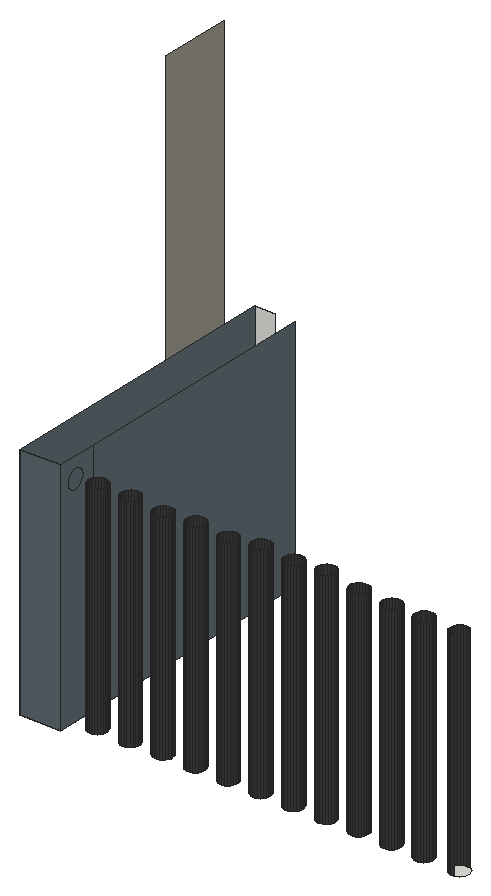
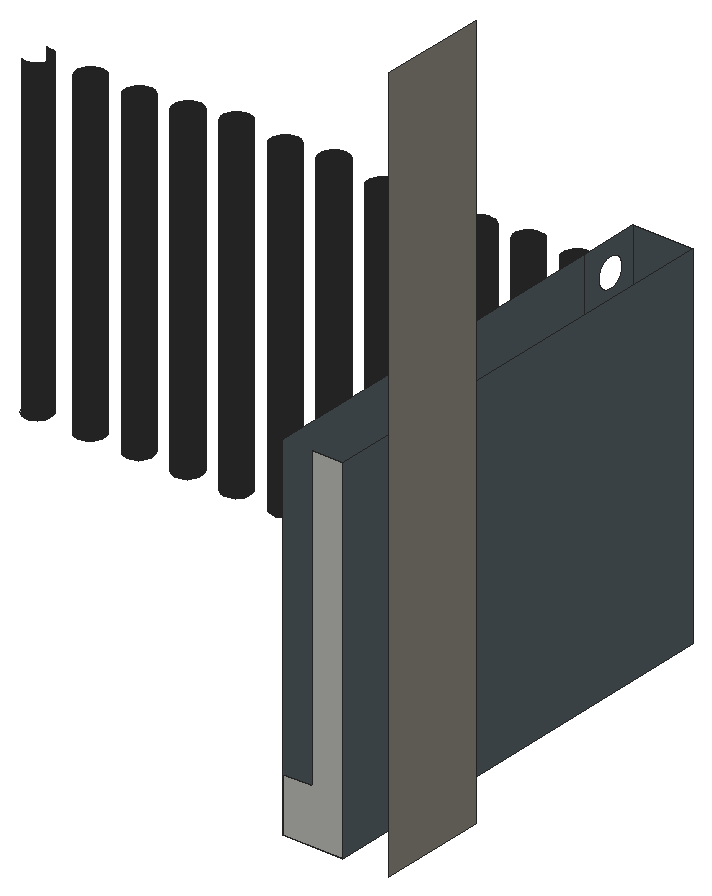
# SketchUp Ruby script. Lengths in inches.
U = 1.inch
M = Sketchup.active_model
def pt(a) = Geom::Point3d.new(a.map { |v| v * U })
def face(e, loops, mat)
  f = e.add_face(loops[0].map { |a| pt(a) })
  loops[1..].each { |l| e.add_face(l.map { |a| pt(a) }).erase! }
  f.material = f.back_material = mat if mat
  f
end
# faces: each face lists its corners as indices into pts; further lists are holes
def faces(e, pts, list, mat = nil) = list.each { |f| face(e, (f[0].is_a?(Array) ? f : [f]).map { |l| l.map { |i| pts[i] } }, mat) }
# xy, xz, yz: faces in a plane at the given z, y or x. An outline is a flat list of corners, or four numbers for a rectangle; further outlines are holes
def ring(l) = l.size == 4 ? [[l[0], l[1]], [l[2], l[1]], [l[2], l[3]], [l[0], l[3]]] : l.each_slice(2).to_a
def flat(e, list, mat, &to3) = list.each { |f| face(e, (f[0].is_a?(Array) ? f : [f]).map { |l| ring(l).map { |u, v| to3.(u, v) } }, mat) }
def xy(e, z, list, mat = nil) = flat(e, list, mat) { |x, y| [x, y, z] }
def xz(e, y, list, mat = nil) = flat(e, list, mat) { |x, z| [x, y, z] }
def yz(e, x, list, mat = nil) = flat(e, list, mat) { |y, z| [x, y, z] }
def lines(e, pts, list) = list.each { |a, b| e.add_line(pt(pts[a]), pt(pts[b])) }
# prism: a flat outline (further loops are holes) pulled along v
def prism(e, loops, v, mat = nil)
  f = face(e, loops, mat); d = Geom::Vector3d.new(v.map { |x| x * U })
  f.pushpull(f.normal.samedirection?(d) ? d.length : -d.length)
end
def box(e, o, s, mat = nil) = prism(e, [[o, [o[0] + s[0], o[1], o[2]], [o[0] + s[0], o[1] + s[1], o[2]], [o[0], o[1] + s[1], o[2]]]], [0, 0, s[2]], mat)
def at(x, y, z, deg = 0) = Geom::Transformation.translation(pt([x, y, z])) * Geom::Transformation.rotation(ORIGIN, Z_AXIS, deg.degrees)
def axes(o, x, y, z) = Geom::Transformation.new([*x, 0, *y, 0, *z, 0, *pt(o).to_a, 1])
def part(name) = M.definitions.add(name)
# library, detail: a bought-in or finely detailed component or shape, given as its bounding box
def library(name, o, s) = part(name).tap { |d| box(d.entities, o, s) }
def detail(e, o, s) = box(e.add_group.entities, o, s)
def put(e, d, t, mat = nil) = e.add_instance(d, t).tap { |i| i.material = mat if mat }
def group(e, t, mat = nil) = e.add_group.tap { |g| g.transformation = t; g.material = mat if mat }.entities
root = M.entities
M.materials.add("[Color M07]").color = [58, 58, 58]
M.materials.add("[Formica Graystone]").color = [149, 146, 135]
M.materials.add("[Formica Speckled Grey]").color = [94, 105, 111]
xy(root,452.9,[[220.36,118.22,223.91,144.04],[225.65,119.22,225.45,119.27,225.26,119.375,225.11,119.52,225,119.71,224.94,119.91,224.94,120.125,225,120.33,225.1,120.51,225.25,120.67,225.43,120.77,225.63,120.83,225.85,120.83,226.05,120.78,226.24,120.68,226.39,120.53,226.5,120.35,226.55,120.14,226.56,119.93,226.5,119.72,226.4,119.54,226.25,119.39,226.07,119.28,225.86,119.22],[228.53,119.22,228.32,119.27,228.14,119.375,227.98,119.52,227.875,119.71,227.82,119.91,227.82,120.125,227.87,120.33,227.97,120.51,228.12,120.67,228.3,120.77,228.51,120.83,228.72,120.83,228.93,120.78,229.11,120.68,229.26,120.53,229.37,120.35,229.43,120.14,229.43,119.93,229.38,119.72,229.27,119.54,229.125,119.39,228.94,119.28,228.74,119.22],[231.4,119.22,231.2,119.27,231.01,119.375,230.86,119.52,230.75,119.71,230.69,119.91,230.69,120.125,230.75,120.33,230.85,120.51,231,120.67,231.18,120.77,231.38,120.83,231.6,120.83,231.8,120.78,231.99,120.68,232.14,120.53,232.25,120.35,232.3,120.14,232.31,119.93,232.25,119.72,232.15,119.54,232,119.39,231.82,119.28,231.61,119.22],[234.28,119.22,234.07,119.27,233.89,119.375,233.73,119.52,233.625,119.71,233.57,119.91,233.57,120.125,233.62,120.33,233.72,120.51,233.87,120.67,234.05,120.77,234.26,120.83,234.47,120.83,234.68,120.78,234.86,120.68,235.01,120.53,235.12,120.35,235.18,120.14,235.18,119.93,235.13,119.72,235.02,119.54,234.875,119.39,234.69,119.28,234.49,119.22],
  [237.15,119.22,236.95,119.27,236.76,119.375,236.61,119.52,236.5,119.71,236.44,119.91,236.44,120.125,236.5,120.33,236.6,120.51,236.75,120.67,236.93,120.77,237.13,120.83,237.35,120.83,237.55,120.78,237.74,120.68,237.89,120.53,238,120.35,238.05,120.14,238.06,119.93,238,119.72,237.9,119.54,237.75,119.39,237.57,119.28,237.36,119.22],[240.03,119.22,239.82,119.27,239.64,119.375,239.48,119.52,239.375,119.71,239.32,119.91,239.32,120.125,239.37,120.33,239.47,120.51,239.62,120.67,239.8,120.77,240.01,120.83,240.22,120.83,240.43,120.78,240.61,120.68,240.76,120.53,240.87,120.35,240.93,120.14,240.93,119.93,240.88,119.72,240.77,119.54,240.625,119.39,240.44,119.28,240.24,119.22],[242.9,119.22,242.7,119.27,242.51,119.375,242.36,119.52,242.25,119.71,242.19,119.91,242.19,120.125,242.25,120.33,242.35,120.51,242.5,120.67,242.68,120.77,242.88,120.83,243.1,120.83,243.3,120.78,243.49,120.68,243.64,120.53,243.75,120.35,243.8,120.14,243.81,119.93,243.75,119.72,243.65,119.54,243.5,119.39,243.32,119.28,243.11,119.22],[245.78,119.22,245.57,119.27,245.39,119.375,245.23,119.52,245.125,119.71,245.07,119.91,245.07,120.125,245.12,120.33,245.22,120.51,245.37,120.67,245.55,120.77,245.76,120.83,245.97,120.83,246.18,120.78,246.36,120.68,246.51,120.53,246.62,120.35,246.68,120.14,246.68,119.93,246.63,119.72,246.52,119.54,246.375,119.39,246.19,119.28,245.99,119.22],[248.65,119.22,248.45,119.27,248.26,119.375,248.11,119.52,248,119.71,247.94,119.91,247.94,120.125,248,120.33,248.1,120.51,248.25,120.67,248.43,120.77,248.63,120.83,248.85,120.83,249.05,120.78,249.24,120.68,249.39,120.53,249.5,120.35,249.55,120.14,249.56,119.93,249.5,119.72,249.4,119.54,249.25,119.39,249.07,119.28,248.86,119.22],
  [251.53,119.22,251.32,119.27,251.14,119.375,250.98,119.52,250.875,119.71,250.82,119.91,250.82,120.125,250.87,120.33,250.97,120.51,251.12,120.67,251.3,120.77,251.51,120.83,251.72,120.83,251.93,120.78,252.11,120.68,252.26,120.53,252.37,120.35,252.43,120.14,252.43,119.93,252.38,119.72,252.27,119.54,252.125,119.39,251.94,119.28,251.74,119.22],[254.4,119.22,254.2,119.27,254.01,119.375,253.86,119.52,253.75,119.71,253.69,119.91,253.69,120.125,253.75,120.33,253.85,120.51,254,120.67,254.18,120.77,254.38,120.83,254.6,120.83,254.8,120.78,254.99,120.68,255.14,120.53,255.25,120.35,255.3,120.14,255.31,119.93,255.25,119.72,255.15,119.54,255,119.39,254.82,119.28,254.61,119.22],[257.53,119.22,257.32,119.27,257.14,119.375,256.98,119.52,256.875,119.71,256.82,119.91,256.82,120.125,256.87,120.33,256.97,120.51,257.12,120.67,257.3,120.77,257.51,120.83,257.72,120.83,257.93,120.78,258.11,120.68,258.26,120.53,258.37,120.35,258.43,120.14,258.43,119.93,258.38,119.72,258.27,119.54,258.125,119.39,257.94,119.28,257.74,119.22]])
xz(root,118.22,[[220.36,452.9,223.91,473.83]],"[Formica Speckled Grey]")
xz(root,119.22,[[225.65,452.9,225.86,472.27],[228.53,452.9,228.74,472.27],[231.4,452.9,231.61,472.05],[234.28,452.9,234.49,472.27],[237.15,452.9,237.36,472.05],
  [240.03,452.9,240.24,472.48],[242.9,452.9,243.11,472.27],[245.78,452.9,245.99,472.48],[248.65,452.9,248.86,472.05],[251.53,452.9,251.74,471.82],
  [254.4,452.9,254.61,471.82],[257.53,452.9,257.74,471.82]],"[Color M07]")
xz(root,120.83,[[225.63,452.9,225.85,472.27],[228.51,452.9,228.72,472.27],[231.38,452.9,231.6,472.05],[234.26,452.9,234.47,472.27],[237.13,452.9,237.35,472.05],
  [240.01,452.9,240.22,472.48],[242.88,452.9,243.1,472.27],[245.76,452.9,245.97,472.48],[248.63,452.9,248.85,472.05],[251.51,452.9,251.72,471.82],
  [254.38,452.9,254.6,471.82],[257.51,452.9,257.72,471.82]],"[Color M07]")
xz(root,144.04,[[220.36,452.9,223.91,452.9,223.91,456.09,222.16,456.09,222.16,473.83,220.36,473.83]])
yz(root,217.65,[[137.66,452.9,144.04,495.41]],"[Formica Graystone]")
yz(root,220.36,[[118.22,452.9,144.04,473.83]],"[Formica Speckled Grey]")
yz(root,223.91,[[[118.22,452.9,121.78,473.83],[119.86,471.17,119.64,471.2,119.42,471.29,119.24,471.43,119.1,471.61,119.02,471.82,118.99,472.05,119.02,472.27,119.1,472.48,119.24,472.67,119.42,472.81,119.64,472.89,119.86,472.92,120.09,472.89,120.3,472.81,120.48,472.67,120.62,472.48,120.71,472.27,120.74,472.05,120.71,471.82,120.62,471.61,120.48,471.43,120.3,471.29,120.09,471.2]],[121.78,452.9,144.04,473.83]],"[Formica Speckled Grey]")
yz(root,224.94,[[119.91,452.9,120.125,472.27]],"[Color M07]")
yz(root,227.82,[[119.91,452.9,120.125,472.27]],"[Color M07]")
yz(root,229.43,[[119.93,452.9,120.14,472.27]],"[Color M07]")
yz(root,230.69,[[119.91,452.9,120.125,472.05]],"[Color M07]")
yz(root,233.57,[[119.91,452.9,120.125,472.27]],"[Color M07]")
yz(root,235.18,[[119.93,452.9,120.14,472.27]],"[Color M07]")
yz(root,236.44,[[119.91,452.9,120.125,472.05]],"[Color M07]")
yz(root,239.32,[[119.91,452.9,120.125,472.48]],"[Color M07]")
yz(root,240.93,[[119.93,452.9,120.14,472.48]],"[Color M07]")
yz(root,242.19,[[119.91,452.9,120.125,472.27]],"[Color M07]")
yz(root,245.07,[[119.91,452.9,120.125,472.48]],"[Color M07]")
yz(root,246.68,[[119.93,452.9,120.14,472.48]],"[Color M07]")
yz(root,247.94,[[119.91,452.9,120.125,472.05]],"[Color M07]")
yz(root,250.82,[[119.91,452.9,120.125,471.82]],"[Color M07]")
yz(root,252.43,[[119.93,452.9,120.14,471.82]],"[Color M07]")
yz(root,253.69,[[119.91,452.9,120.125,471.82]],"[Color M07]")
yz(root,256.82,[[119.91,452.9,120.125,471.82]],"[Color M07]")
p = [[225.45,119.27,452.9],[225.65,119.22,452.9],[225.65,119.22,472.27],[225.45,119.27,472.27],[225.86,119.22,452.9],[226.07,119.28,452.9],
  [226.07,119.28,472.27],[225.86,119.22,472.27],[228.32,119.27,452.9],[228.53,119.22,452.9],[228.53,119.22,472.27],[228.32,119.27,472.27],
  [228.74,119.22,452.9],[228.94,119.28,452.9],[228.94,119.28,472.27],[228.74,119.22,472.27],[231.2,119.27,452.9],[231.4,119.22,452.9],
  [231.4,119.22,472.05],[231.2,119.27,472.05],[231.61,119.22,452.9],[231.82,119.28,452.9],[231.82,119.28,472.05],[231.61,119.22,472.05],
  [234.07,119.27,452.9],[234.28,119.22,452.9],[234.28,119.22,472.27],[234.07,119.27,472.27],[234.49,119.22,452.9],[234.69,119.28,452.9],
  [234.69,119.28,472.27],[234.49,119.22,472.27],[236.95,119.27,452.9],[237.15,119.22,452.9],[237.15,119.22,472.05],[236.95,119.27,472.05],
  [237.36,119.22,452.9],[237.57,119.28,452.9],[237.57,119.28,472.05],[237.36,119.22,472.05],[239.82,119.27,452.9],[240.03,119.22,452.9],
  [240.03,119.22,472.48],[239.82,119.27,472.48],[240.24,119.22,452.9],[240.44,119.28,452.9],[240.44,119.28,472.48],[240.24,119.22,472.48],
  [242.7,119.27,452.9],[242.9,119.22,452.9],[242.9,119.22,472.27],[242.7,119.27,472.27],[243.11,119.22,452.9],[243.32,119.28,452.9],
  [243.32,119.28,472.27],[243.11,119.22,472.27],[245.57,119.27,452.9],[245.78,119.22,452.9],[245.78,119.22,472.48],[245.57,119.27,472.48],
  [245.99,119.22,452.9],[246.19,119.28,452.9],[246.19,119.28,472.48],[245.99,119.22,472.48],[248.45,119.27,452.9],[248.65,119.22,452.9],
  [248.65,119.22,472.05],[248.45,119.27,472.05],[248.86,119.22,452.9],[249.07,119.28,452.9],[249.07,119.28,472.05],[248.86,119.22,472.05],
  [251.32,119.27,452.9],[251.53,119.22,452.9],[251.53,119.22,471.82],[251.32,119.27,471.82],[251.74,119.22,452.9],[251.94,119.28,452.9],
  [251.94,119.28,471.82],[251.74,119.22,471.82],[254.2,119.27,452.9],[254.4,119.22,452.9],[254.4,119.22,471.82],[254.2,119.27,471.82],
  [254.61,119.22,452.9],[254.82,119.28,452.9],[254.82,119.28,471.82],[254.61,119.22,471.82],[257.32,119.27,452.9],[257.53,119.22,452.9],
  [257.53,119.22,471.82],[257.32,119.27,471.82],[225.26,119.375,452.9],[225.26,119.375,472.27],[226.25,119.39,452.9],[226.25,119.39,472.27],
  [228.14,119.375,452.9],[228.14,119.375,472.27],[229.125,119.39,452.9],[229.125,119.39,472.27],[231.01,119.375,452.9],[231.01,119.375,472.05],
  [232,119.39,452.9],[232,119.39,472.05],[233.89,119.375,452.9],[233.89,119.375,472.27],[234.875,119.39,452.9],[234.875,119.39,472.27],
  [236.76,119.375,452.9],[236.76,119.375,472.05],[237.75,119.39,452.9],[237.75,119.39,472.05],[239.64,119.375,452.9],[239.64,119.375,472.48],
  [240.625,119.39,452.9],[240.625,119.39,472.48],[242.51,119.375,452.9],[242.51,119.375,472.27],[243.5,119.39,452.9],[243.5,119.39,472.27],
  [245.39,119.375,452.9],[245.39,119.375,472.48],[246.375,119.39,452.9],[246.375,119.39,472.48],[248.26,119.375,452.9],[248.26,119.375,472.05],
  [249.25,119.39,452.9],[249.25,119.39,472.05],[251.14,119.375,452.9],[251.14,119.375,471.82],[252.125,119.39,452.9],[252.125,119.39,471.82],
  [254.01,119.375,452.9],[254.01,119.375,471.82],[255,119.39,452.9],[255,119.39,471.82],[257.14,119.375,452.9],[257.14,119.375,471.82],
  [225.11,119.52,452.9],[225.11,119.52,472.27],[226.4,119.54,452.9],[226.4,119.54,472.27],[227.98,119.52,452.9],[227.98,119.52,472.27],
  [229.27,119.54,452.9],[229.27,119.54,472.27],[230.86,119.52,452.9],[230.86,119.52,472.05],[232.15,119.54,452.9],[232.15,119.54,472.05],
  [233.73,119.52,452.9],[233.73,119.52,472.27],[235.02,119.54,452.9],[235.02,119.54,472.27],[236.61,119.52,452.9],[236.61,119.52,472.05],
  [237.9,119.54,452.9],[237.9,119.54,472.05],[239.48,119.52,452.9],[239.48,119.52,472.48],[240.77,119.54,452.9],[240.77,119.54,472.48],
  [242.36,119.52,452.9],[242.36,119.52,472.27],[243.65,119.54,452.9],[243.65,119.54,472.27],[245.23,119.52,452.9],[245.23,119.52,472.48],
  [246.52,119.54,452.9],[246.52,119.54,472.48],[248.11,119.52,452.9],[248.11,119.52,472.05],[249.4,119.54,452.9],[249.4,119.54,472.05],
  [250.98,119.52,452.9],[250.98,119.52,471.82],[252.27,119.54,452.9],[252.27,119.54,471.82],[253.86,119.52,452.9],[253.86,119.52,471.82],
  [255.15,119.54,452.9],[255.15,119.54,471.82],[256.98,119.52,452.9],[256.98,119.52,471.82],[225,119.71,452.9],[225,119.71,472.27],
  [226.5,119.72,452.9],[226.5,119.72,472.27],[227.875,119.71,452.9],[227.875,119.71,472.27],[229.38,119.72,452.9],[229.38,119.72,472.27],
  [230.75,119.71,452.9],[230.75,119.71,472.05],[232.25,119.72,452.9],[232.25,119.72,472.05],[233.625,119.71,452.9],[233.625,119.71,472.27],
  [235.13,119.72,452.9],[235.13,119.72,472.27],[236.5,119.71,452.9],[236.5,119.71,472.05],[238,119.72,452.9],[238,119.72,472.05],
  [239.375,119.71,452.9],[239.375,119.71,472.48],[240.88,119.72,452.9],[240.88,119.72,472.48],[242.25,119.71,452.9],[242.25,119.71,472.27],
  [243.75,119.72,452.9],[243.75,119.72,472.27],[245.125,119.71,452.9],[245.125,119.71,472.48],[246.63,119.72,452.9],[246.63,119.72,472.48],
  [248,119.71,452.9],[248,119.71,472.05],[249.5,119.72,452.9],[249.5,119.72,472.05],[250.875,119.71,452.9],[250.875,119.71,471.82],
  [252.38,119.72,452.9],[252.38,119.72,471.82],[253.75,119.71,452.9],[253.75,119.71,471.82],[255.25,119.72,452.9],[255.25,119.72,471.82],
  [256.875,119.71,452.9],[256.875,119.71,471.82],[224.94,119.91,452.9],[224.94,119.91,472.27],[226.56,119.93,452.9],[226.56,119.93,472.27],
  [227.82,119.91,452.9],[227.82,119.91,472.27],[229.43,119.93,452.9],[229.43,119.93,472.27],[230.69,119.91,452.9],[230.69,119.91,472.05],
  [232.31,119.93,452.9],[232.31,119.93,472.05],[233.57,119.91,452.9],[233.57,119.91,472.27],[235.18,119.93,452.9],[235.18,119.93,472.27],
  [236.44,119.91,452.9],[236.44,119.91,472.05],[238.06,119.93,452.9],[238.06,119.93,472.05],[239.32,119.91,452.9],[239.32,119.91,472.48],
  [240.93,119.93,452.9],[240.93,119.93,472.48],[242.19,119.91,452.9],[242.19,119.91,472.27],[243.81,119.93,452.9],[243.81,119.93,472.27],
  [245.07,119.91,452.9],[245.07,119.91,472.48],[246.68,119.93,452.9],[246.68,119.93,472.48],[247.94,119.91,452.9],[247.94,119.91,472.05],
  [249.56,119.93,452.9],[249.56,119.93,472.05],[250.82,119.91,452.9],[250.82,119.91,471.82],[252.43,119.93,452.9],[252.43,119.93,471.82],
  [253.69,119.91,452.9],[253.69,119.91,471.82],[255.31,119.93,452.9],[255.31,119.93,471.82],[256.82,119.91,452.9],[256.82,119.91,471.82],
  [226.55,120.14,452.9],[226.55,120.14,472.27],[232.3,120.14,452.9],[232.3,120.14,472.05],[238.05,120.14,452.9],[238.05,120.14,472.05],
  [243.8,120.14,452.9],[243.8,120.14,472.27],[249.55,120.14,452.9],[249.55,120.14,472.05],[255.3,120.14,452.9],[255.3,120.14,471.82],
  [225,120.33,452.9],[224.94,120.125,452.9],[224.94,120.125,472.27],[225,120.33,472.27],[226.5,120.35,452.9],[226.5,120.35,472.27],
  [227.87,120.33,452.9],[227.82,120.125,452.9],[227.82,120.125,472.27],[227.87,120.33,472.27],[229.43,120.14,452.9],[229.37,120.35,452.9],
  [229.37,120.35,472.27],[229.43,120.14,472.27],[230.75,120.33,452.9],[230.69,120.125,452.9],[230.69,120.125,472.05],[230.75,120.33,472.05],
  [232.25,120.35,452.9],[232.25,120.35,472.05],[233.62,120.33,452.9],[233.57,120.125,452.9],[233.57,120.125,472.27],[233.62,120.33,472.27],
  [235.18,120.14,452.9],[235.12,120.35,452.9],[235.12,120.35,472.27],[235.18,120.14,472.27],[236.5,120.33,452.9],[236.44,120.125,452.9],
  [236.44,120.125,472.05],[236.5,120.33,472.05],[238,120.35,452.9],[238,120.35,472.05],[239.37,120.33,452.9],[239.32,120.125,452.9],
  [239.32,120.125,472.48],[239.37,120.33,472.48],[240.93,120.14,452.9],[240.87,120.35,452.9],[240.87,120.35,472.48],[240.93,120.14,472.48],
  [242.25,120.33,452.9],[242.19,120.125,452.9],[242.19,120.125,472.27],[242.25,120.33,472.27],[243.75,120.35,452.9],[243.75,120.35,472.27],
  [245.12,120.33,452.9],[245.07,120.125,452.9],[245.07,120.125,472.48],[245.12,120.33,472.48],[246.68,120.14,452.9],[246.62,120.35,452.9],
  [246.62,120.35,472.48],[246.68,120.14,472.48],[248,120.33,452.9],[247.94,120.125,452.9],[247.94,120.125,472.05],[248,120.33,472.05],
  [249.5,120.35,452.9],[249.5,120.35,472.05],[250.87,120.33,452.9],[250.82,120.125,452.9],[250.82,120.125,471.82],[250.87,120.33,471.82],
  [252.43,120.14,452.9],[252.37,120.35,452.9],[252.37,120.35,471.82],[252.43,120.14,471.82],[253.75,120.33,452.9],[253.69,120.125,452.9],
  [253.69,120.125,471.82],[253.75,120.33,471.82],[255.25,120.35,452.9],[255.25,120.35,471.82],[256.87,120.33,452.9],[256.82,120.125,452.9],
  [256.82,120.125,471.82],[256.87,120.33,471.82],[225.1,120.51,452.9],[225.1,120.51,472.27],[226.39,120.53,452.9],[226.39,120.53,472.27],
  [227.97,120.51,452.9],[227.97,120.51,472.27],[229.26,120.53,452.9],[229.26,120.53,472.27],[230.85,120.51,452.9],[230.85,120.51,472.05],
  [232.14,120.53,452.9],[232.14,120.53,472.05],[233.72,120.51,452.9],[233.72,120.51,472.27],[235.01,120.53,452.9],[235.01,120.53,472.27],
  [236.6,120.51,452.9],[236.6,120.51,472.05],[237.89,120.53,452.9],[237.89,120.53,472.05],[239.47,120.51,452.9],[239.47,120.51,472.48],
  [240.76,120.53,452.9],[240.76,120.53,472.48],[242.35,120.51,452.9],[242.35,120.51,472.27],[243.64,120.53,452.9],[243.64,120.53,472.27],
  [245.22,120.51,452.9],[245.22,120.51,472.48],[246.51,120.53,452.9],[246.51,120.53,472.48],[248.1,120.51,452.9],[248.1,120.51,472.05],
  [249.39,120.53,452.9],[249.39,120.53,472.05],[250.97,120.51,452.9],[250.97,120.51,471.82],[252.26,120.53,452.9],[252.26,120.53,471.82],
  [253.85,120.51,452.9],[253.85,120.51,471.82],[255.14,120.53,452.9],[255.14,120.53,471.82],[256.97,120.51,452.9],[256.97,120.51,471.82],
  [225.25,120.67,452.9],[225.25,120.67,472.27],[226.24,120.68,452.9],[226.24,120.68,472.27],[228.12,120.67,452.9],[228.12,120.67,472.27],
  [229.11,120.68,452.9],[229.11,120.68,472.27],[231,120.67,452.9],[231,120.67,472.05],[231.99,120.68,452.9],[231.99,120.68,472.05],
  [233.87,120.67,452.9],[233.87,120.67,472.27],[234.86,120.68,452.9],[234.86,120.68,472.27],[236.75,120.67,452.9],[236.75,120.67,472.05],
  [237.74,120.68,452.9],[237.74,120.68,472.05],[239.62,120.67,452.9],[239.58,120.62,472.48],[239.62,120.67,472.48],[240.61,120.68,452.9],
  [240.61,120.68,472.48],[240.67,120.62,472.48],[242.5,120.67,452.9],[242.5,120.67,472.27],[243.49,120.68,452.9],[243.49,120.68,472.27],
  [245.37,120.67,452.9],[245.33,120.62,472.48],[245.37,120.67,472.48],[246.36,120.68,452.9],[246.36,120.68,472.48],[246.42,120.62,472.48],
  [248.25,120.67,452.9],[248.25,120.67,472.05],[249.24,120.68,452.9],[249.24,120.68,472.05],[251.12,120.67,452.9],[251.12,120.67,471.82],
  [252.11,120.68,452.9],[252.11,120.68,471.82],[254,120.67,452.9],[254,120.67,471.82],[254.99,120.68,452.9],[254.99,120.68,471.82],
  [257.12,120.67,452.9],[257.12,120.67,471.82],[225.43,120.77,452.9],[225.32,120.71,472.27],[225.43,120.77,472.27],[226.05,120.78,452.9],
  [226.05,120.78,472.27],[226.18,120.71,472.27],[228.3,120.77,452.9],[228.19,120.71,472.27],[228.3,120.77,472.27],[228.93,120.78,452.9],
  [228.93,120.78,472.27],[229.06,120.71,472.27],[231.18,120.77,452.9],[231.12,120.74,472.05],[231.18,120.77,472.05],[231.8,120.78,452.9],
  [231.8,120.78,472.05],[231.88,120.74,472.05],[234.05,120.77,452.9],[233.94,120.71,472.27],[234.05,120.77,472.27],[234.68,120.78,452.9],
  [234.68,120.78,472.27],[234.81,120.71,472.27],[236.93,120.77,452.9],[236.87,120.74,472.05],[236.93,120.77,472.05],[237.55,120.78,452.9],
  [237.55,120.78,472.05],[237.63,120.74,472.05],[239.8,120.77,452.9],[239.8,120.77,472.48],[240.43,120.78,452.9],[240.43,120.78,472.48],
  [242.68,120.77,452.9],[242.57,120.71,472.27],[242.68,120.77,472.27],[243.3,120.78,452.9],[243.3,120.78,472.27],[243.43,120.71,472.27],
  [245.55,120.77,452.9],[245.55,120.77,472.48],[246.18,120.78,452.9],[246.18,120.78,472.48],[248.43,120.77,452.9],[248.37,120.74,472.05],
  [248.43,120.77,472.05],[249.05,120.78,452.9],[249.05,120.78,472.05],[249.13,120.74,472.05],[251.3,120.77,452.9],[251.19,120.71,471.82],
  [251.3,120.77,471.82],[251.93,120.78,452.9],[251.93,120.78,471.82],[252.06,120.71,471.82],[254.18,120.77,452.9],[254.07,120.71,471.82],
  [254.18,120.77,471.82],[254.8,120.78,452.9],[254.8,120.78,471.82],[254.93,120.71,471.82],[257.3,120.77,452.9],[257.19,120.71,471.82],
  [257.3,120.77,471.82],[225.63,120.83,452.9],[225.63,120.83,472.27],[225.85,120.83,452.9],[225.85,120.83,472.27],[228.51,120.83,452.9],
  [228.51,120.83,472.27],[228.72,120.83,452.9],[228.72,120.83,472.27],[231.38,120.83,452.9],[231.38,120.83,472.05],[231.6,120.83,452.9],
  [231.6,120.83,472.05],[234.26,120.83,452.9],[234.26,120.83,472.27],[234.47,120.83,452.9],[234.47,120.83,472.27],[237.13,120.83,452.9],
  [237.13,120.83,472.05],[237.35,120.83,452.9],[237.35,120.83,472.05],[240.01,120.83,452.9],[240.01,120.83,472.48],[240.22,120.83,452.9],
  [240.22,120.83,472.48],[242.88,120.83,452.9],[242.88,120.83,472.27],[243.1,120.83,452.9],[243.1,120.83,472.27],[245.76,120.83,452.9],
  [245.76,120.83,472.48],[245.97,120.83,452.9],[245.97,120.83,472.48],[248.63,120.83,452.9],[248.63,120.83,472.05],[248.85,120.83,452.9],
  [248.85,120.83,472.05],[251.51,120.83,452.9],[251.51,120.83,471.82],[251.72,120.83,452.9],[251.72,120.83,471.82],[254.38,120.83,452.9],
  [254.38,120.83,471.82],[254.6,120.83,452.9],[254.6,120.83,471.82],[257.51,120.83,452.9],[257.51,120.83,471.82],[257.93,120.78,452.9],
  [257.72,120.83,452.9],[257.72,120.83,471.82],[257.93,120.78,471.82]]
faces(root,p,[[0,1,2,3],[4,5,6,7],[8,9,10,11],[12,13,14,15],[16,17,18,19],[20,21,22,23],[24,25,26,27],[28,29,30,31],
  [32,33,34,35],[36,37,38,39],[40,41,42,43],[44,45,46,47],[48,49,50,51],[52,53,54,55],[56,57,58,59],[60,61,62,63],
  [64,65,66,67],[68,69,70,71],[72,73,74,75],[76,77,78,79],[80,81,82,83],[84,85,86,87],[88,89,90,91],[92,0,3,93],
  [5,94,95,6],[96,8,11,97],[13,98,99,14],[100,16,19,101],[21,102,103,22],[104,24,27,105],[29,106,107,30],[108,32,35,109],
  [37,110,111,38],[112,40,43,113],[45,114,115,46],[116,48,51,117],[53,118,119,54],[120,56,59,121],[61,122,123,62],[124,64,67,125],
  [69,126,127,70],[128,72,75,129],[77,130,131,78],[132,80,83,133],[85,134,135,86],[136,88,91,137],[138,92,93,139],[94,140,141,95],
  [142,96,97,143],[98,144,145,99],[146,100,101,147],[102,148,149,103],[150,104,105,151],[106,152,153,107],[154,108,109,155],[110,156,157,111],
  [158,112,113,159],[114,160,161,115],[162,116,117,163],[118,164,165,119],[166,120,121,167],[122,168,169,123],[170,124,125,171],[126,172,173,127],
  [174,128,129,175],[130,176,177,131],[178,132,133,179],[134,180,181,135],[182,136,137,183],[184,138,139,185],[140,186,187,141],[188,142,143,189],
  [144,190,191,145],[192,146,147,193],[148,194,195,149],[196,150,151,197],[152,198,199,153],[200,154,155,201],[156,202,203,157],[204,158,159,205],
  [160,206,207,161],[208,162,163,209],[164,210,211,165],[212,166,167,213],[168,214,215,169],[216,170,171,217],[172,218,219,173],[220,174,175,221],
  [176,222,223,177],[224,178,179,225],[180,226,227,181],[228,182,183,229],[230,184,185,231],[186,232,233,187],[234,188,189,235],[190,236,237,191],
  [238,192,193,239],[194,240,241,195],[242,196,197,243],[198,244,245,199],[246,200,201,247],[202,248,249,203],[250,204,205,251],[206,252,253,207],
  [254,208,209,255],[210,256,257,211],[258,212,213,259],[214,260,261,215],[262,216,217,263],[218,264,265,219],[266,220,221,267],[222,268,269,223],
  [270,224,225,271],[226,272,273,227],[274,228,229,275],[232,276,277,233],[240,278,279,241],[248,280,281,249],[256,282,283,257],[264,284,285,265],
  [272,286,287,273],[288,289,290,291],[276,292,293,277],[294,295,296,297],[298,299,300,301],[302,303,304,305],[278,306,307,279],[308,309,310,311],
  [312,313,314,315],[316,317,318,319],[280,320,321,281],[322,323,324,325],[326,327,328,329],[330,331,332,333],[282,334,335,283],[336,337,338,339],
  [340,341,342,343],[344,345,346,347],[284,348,349,285],[350,351,352,353],[354,355,356,357],[358,359,360,361],[286,362,363,287],[364,365,366,367],
  [368,288,291,369],[292,370,371,293],[372,294,297,373],[299,374,375,300],[376,302,305,377],[306,378,379,307],[380,308,311,381],[313,382,383,314],
  [384,316,319,385],[320,386,387,321],[388,322,325,389],[327,390,391,328],[392,330,333,393],[334,394,395,335],[396,336,339,397],[341,398,399,342],
  [400,344,347,401],[348,402,403,349],[404,350,353,405],[355,406,407,356],[408,358,361,409],[362,410,411,363],[412,364,367,413],[414,368,369,415],
  [370,416,417,371],[418,372,373,419],[374,420,421,375],[422,376,377,423],[378,424,425,379],[426,380,381,427],[382,428,429,383],[430,384,385,431],
  [386,432,433,387],[434,388,389,435,436],[390,437,438,439,391],[440,392,393,441],[394,442,443,395],[444,396,397,445,446],[398,447,448,449,399],[450,400,401,451],
  [402,452,453,403],[454,404,405,455],[406,456,457,407],[458,408,409,459],[410,460,461,411],[462,412,413,463],[464,414,415,465,466],[416,467,468,469,417],
  [470,418,419,471,472],[420,473,474,475,421],[476,422,423,477,478],[424,479,480,481,425],[482,426,427,483,484],[428,485,486,487,429],[488,430,431,489,490],[432,491,492,493,433],
  [494,434,436,495],[437,496,497,438],[498,440,441,499,500],[442,501,502,503,443],[504,444,446,505],[447,506,507,448],[508,450,451,509,510],[452,511,512,513,453],
  [514,454,455,515,516],[456,517,518,519,457],[520,458,459,521,522],[460,523,524,525,461],[526,462,463,527,528],[529,464,466,530],[467,531,532,468],[533,470,472,534],
  [473,535,536,474],[537,476,478,538],[479,539,540,480],[541,482,484,542],[485,543,544,486],[545,488,490,546],[491,547,548,492],[549,494,495,550],
  [496,551,552,497],[553,498,500,554],[501,555,556,502],[557,504,505,558],[506,559,560,507],[561,508,510,562],[511,563,564,512],[565,514,516,566],
  [517,567,568,518],[569,520,522,570],[523,571,572,524],[573,526,528,574],[575,576,577,578]],"[Color M07]")
